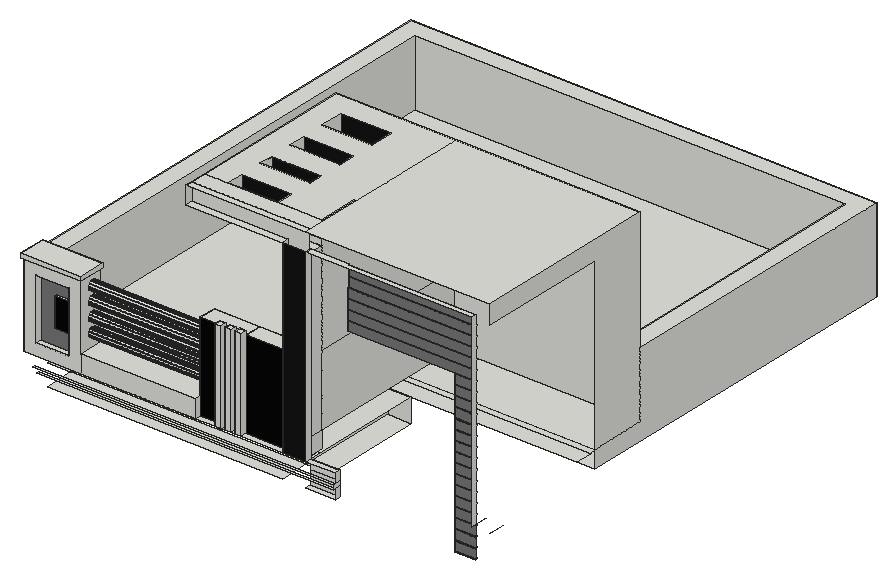
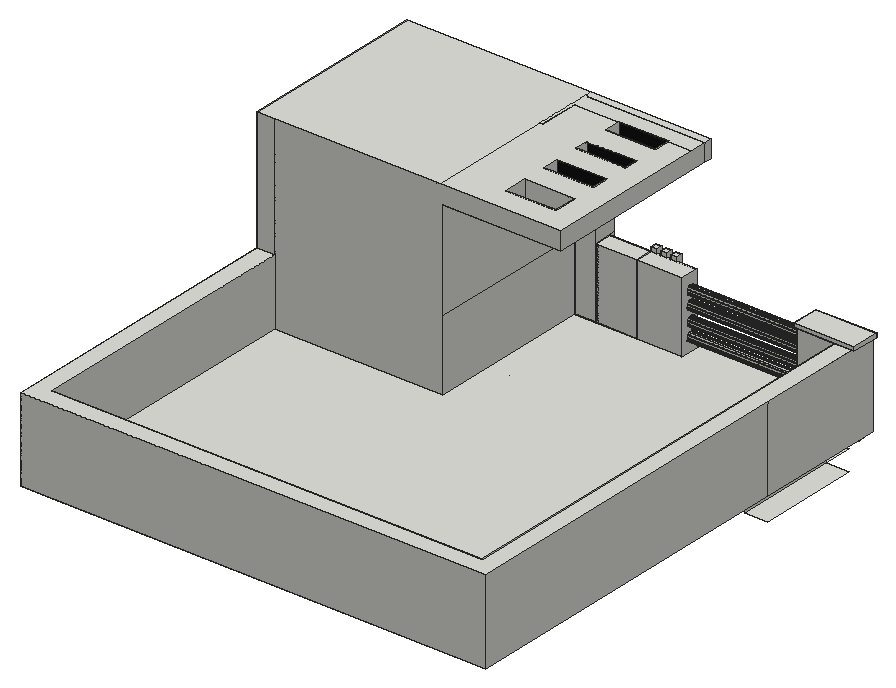
# SketchUp Ruby script. Lengths in inches.
U = 1.inch
M = Sketchup.active_model
def pt(a) = Geom::Point3d.new(a.map { |v| v * U })
def face(e, loops, mat)
  f = e.add_face(loops[0].map { |a| pt(a) })
  loops[1..].each { |l| e.add_face(l.map { |a| pt(a) }).erase! }
  f.material = f.back_material = mat if mat
  f
end
# faces: each face lists its corners as indices into pts; further lists are holes
def faces(e, pts, list, mat = nil) = list.each { |f| face(e, (f[0].is_a?(Array) ? f : [f]).map { |l| l.map { |i| pts[i] } }, mat) }
# xy, xz, yz: faces in a plane at the given z, y or x. An outline is a flat list of corners, or four numbers for a rectangle; further outlines are holes
def ring(l) = l.size == 4 ? [[l[0], l[1]], [l[2], l[1]], [l[2], l[3]], [l[0], l[3]]] : l.each_slice(2).to_a
def flat(e, list, mat, &to3) = list.each { |f| face(e, (f[0].is_a?(Array) ? f : [f]).map { |l| ring(l).map { |u, v| to3.(u, v) } }, mat) }
def xy(e, z, list, mat = nil) = flat(e, list, mat) { |x, y| [x, y, z] }
def xz(e, y, list, mat = nil) = flat(e, list, mat) { |x, z| [x, y, z] }
def yz(e, x, list, mat = nil) = flat(e, list, mat) { |y, z| [x, y, z] }
def lines(e, pts, list) = list.each { |a, b| e.add_line(pt(pts[a]), pt(pts[b])) }
# prism: a flat outline (further loops are holes) pulled along v
def prism(e, loops, v, mat = nil)
  f = face(e, loops, mat); d = Geom::Vector3d.new(v.map { |x| x * U })
  f.pushpull(f.normal.samedirection?(d) ? d.length : -d.length)
end
def box(e, o, s, mat = nil) = prism(e, [[o, [o[0] + s[0], o[1], o[2]], [o[0] + s[0], o[1] + s[1], o[2]], [o[0], o[1] + s[1], o[2]]]], [0, 0, s[2]], mat)
def at(x, y, z, deg = 0) = Geom::Transformation.translation(pt([x, y, z])) * Geom::Transformation.rotation(ORIGIN, Z_AXIS, deg.degrees)
def axes(o, x, y, z) = Geom::Transformation.new([*x, 0, *y, 0, *z, 0, *pt(o).to_a, 1])
def part(name) = M.definitions.add(name)
# library, detail: a bought-in or finely detailed component or shape, given as its bounding box
def library(name, o, s) = part(name).tap { |d| box(d.entities, o, s) }
def detail(e, o, s) = box(e.add_group.entities, o, s)
def put(e, d, t, mat = nil) = e.add_instance(d, t).tap { |i| i.material = mat if mat }
def group(e, t, mat = nil) = e.add_group.tap { |g| g.transformation = t; g.material = mat if mat }.entities
root = M.entities
M.materials.add("[0135_DarkGray]1").color = [119, 119, 119]
M.materials.add("[0136_Charcoal]").color = [7, 7, 7]
M.materials.add("[0136_Charcoal]1").color = [20, 20, 20]
xy(root,232.85,[[219.1875,3.625,229.75,4.125]])
xy(root,233.35,[[219.1875,3.625,229.75,4.125]])
xy(root,237,[[13,1.125,133.04,16.125],[145.04,1.125,160.04,4.125],[133.04,16.125,145.04,68.1875]])
xy(root,237.0625,[[1,16.125,12.875,68.1875]])
xy(root,237.93,[[219.1875,3.625,229.75,4.125]])
xy(root,238.43,[[219.1875,3.625,229.75,4.125]])
xy(root,242,[[8.5,0.125,160.04,1.125]])
xy(root,243,[[219.1875,3.625,229.75,4.125]])
xy(root,243.5,[[219.1875,3.625,229.75,4.125]])
xy(root,244,[[6.5,0.125,160.04,1.125]])
xy(root,248.08,[[219.1875,3.625,229.75,4.125]])
xy(root,248.58,[[219.1875,3.625,229.75,4.125]])
xy(root,249,[[1,1.125,12.875,68.1875],[12.875,1.125,12.875,16.125,133.04,16.125,133.04,13.125,111.875,13.125,111.875,1.125,108.875,1.125,108.875,4.125,106.8125,4.125,106.8125,1.125,103.8125,1.125,103.8125,4.125,101.6875,4.125,101.6875,1.125,98.6875,1.125,98.6875,4.125,88.625,4.125,88.625,1.125],[88.625,1.125,98.6875,4.125],[101.6875,1.125,103.8125,4.125],[106.8125,1.125,108.875,4.125],
  [111.875,1.125,133.04,4.125],[133.04,1.125,143.7,10.125],[145.04,1.125,160.04,4.125],[111.875,4.125,133.04,13.125],[145.04,4.125,143.7,4.87,143.7,10.125,145.04,10.125],
  [133.04,10.125,143.7,13.125],[143.7,10.125,143.7,13.125,133.04,13.125,133.04,68.1875,145.04,68.1875,145.04,10.125],[12.875,16.125,133.04,68.1875],[1,68.1875,229.75,68.1875,229.75,77.1875,10,77.1875,10,239.1875,229.75,239.1875,229.75,248.1875,1,248.1875],[229.75,68.1875,238.75,248.1875],
  [10,77.1875,229.75,239.1875]])
xy(root,253.15,[[219.1875,3.625,229.75,4.125]])
xy(root,253.65,[[219.1875,3.625,229.75,4.125]])
xy(root,255,[[7,1.125,24,4.125]])
xy(root,258,[[30,1.125,88.625,1.125,88.625,13.125,143.7,13.125,143.7,97.125,229.75,97.125,229.75,239.1875,10,239.1875,10,13.125,30,13.125]])
xy(root,258.23,[[219.1875,3.625,229.75,4.125]])
xy(root,258.73,[[219.1875,3.625,229.75,4.125]])
xy(root,263.3,[[219.1875,3.625,229.75,4.125]])
xy(root,263.8,[[219.1875,3.625,229.75,4.125]])
xy(root,264,[[15.5,2.625,24,4.125]])
xy(root,268.375,[[219.1875,3.625,229.75,4.125]])
xy(root,268.875,[[219.1875,3.625,229.75,4.125]])
xy(root,273.45,[[219.1875,3.625,229.75,4.125]])
xy(root,273.95,[[219.1875,3.625,229.75,4.125]])
xy(root,278.53,[[219.1875,3.625,229.75,4.125]])
xy(root,278.5625,[[15.5,2.625,24,4.125]])
xy(root,279.03,[[219.1875,3.625,229.75,4.125]])
xy(root,283.6,[[219.1875,3.625,229.75,4.125]])
xy(root,284.1,[[219.1875,3.625,229.75,4.125]])
xy(root,286,[[7,1.125,24,4.125]])
xy(root,288.68,[[219.1875,3.625,229.75,4.125]])
xy(root,289.18,[[219.1875,3.625,229.75,4.125]])
xy(root,292,[[0,0,31,1.125],[0,1.125,1,13.125],[1,1.125,30,13.125],[30,1.125,31,4.125],[30,4.125,31,14.125],
  [0,13.125,1,14.125],[1,13.125,10,14.125],[10,13.125,30,14.125],[1,14.125,10,14.125,10,239.1875,229.75,239.1875,229.75,97.125,238.75,97.125,238.75,248.1875,1,248.1875]])
xy(root,293.75,[[219.1875,3.625,229.75,4.125]])
xy(root,294,[[0,0,31,14.125],[88.625,4.125,111.875,13.125],[111.875,4.125,132.95,13.125]])
xy(root,294.25,[[219.1875,3.625,229.75,4.125]])
xy(root,296,[[98.6875,1.125,101.6875,4.125],[103.8125,1.125,106.8125,4.125],[108.875,1.125,111.875,4.125]])
xy(root,298.83,[[219.1875,3.625,229.75,4.125]])
xy(root,299.33,[[219.1875,3.625,229.75,4.125]])
xy(root,303.9,[[219.1875,3.625,229.75,4.125]])
xy(root,304.4,[[219.1875,3.625,229.75,4.125]])
xy(root,308.98,[[219.1875,3.625,229.75,4.125]])
xy(root,309.48,[[219.1875,3.625,229.75,4.125]])
xy(root,314.05,[[219.1875,3.625,229.75,4.125]])
xy(root,314.55,[[164.62,3.625,229.75,4.125]])
xy(root,319.125,[[164.62,3.625,229.75,4.125]])
xy(root,319.625,[[164.62,3.625,229.75,4.125]])
xy(root,324.2,[[164.62,3.625,229.75,4.125]])
xy(root,324.7,[[164.62,3.625,229.75,4.125]])
xy(root,329.28,[[164.62,3.625,229.75,4.125]])
xy(root,329.78,[[164.62,3.625,229.75,4.125]])
xy(root,334.35,[[164.62,3.625,229.75,4.125]])
xy(root,334.85,[[164.62,3.6875,229.75,4.125]])
xy(root,339.43,[[164.62,3.6875,229.75,4.125]])
xy(root,339.93,[[164.62,3.6875,229.75,4.125]])
xy(root,342,[[132.95,4.87,143.7,13.125]])
xy(root,345,[[83.7,1.125,132.95,4.87],[145.04,1.125,145.04,4.125,164.62,4.125,164.62,3.6875,229.75,3.6875,229.75,1.125],[[83.7,4.87,83.7,97.125,143.7,97.125,143.7,13.125,132.95,13.125,132.95,4.87],[95.7,13.125,121.04,85.125]]])
xy(root,345,[[95.7,21.5625,121.04,33.5625],[95.7,40.66,121.04,52.66],[95.7,61.125,121.04,73.125]],"[0136_Charcoal]1")
xy(root,354,[[83.7,1.125,145.04,1.125,145.04,4.125,143.7,4.87,83.7,4.87],[145.04,1.125,238.75,97.125],[145.04,4.125,145.04,33.5625,143.7,33.5625,143.7,13.125,83.7,13.125,83.7,4.87,143.7,4.87],[[83.7,13.125,95.7,13.125,95.7,21.5625,121.04,21.5625,121.04,13.125,143.7,13.125,143.7,33.5625,145.04,33.5625,145.04,97.125,83.7,97.125],[95.7,73.125,121.04,85.125],[95.7,52.66,121.04,61.125],[95.7,33.5625,121.04,40.66]]])
xz(root,0,[[0,292,31,294]])
xz(root,1.125,[[[1,249,30,292],[7,255,24,286]],[30,249,88.625,258],[98.6875,249,101.6875,296],[103.8125,249,106.8125,296],[108.875,249,111.875,296]])
xz(root,1.125,[[133.04,249,145.04,249,145.04,345,132.95,345,132.95,294]],"[0136_Charcoal]1")
xz(root,2.625,[[15.5,264,24,278.5625]],"[0136_Charcoal]")
xz(root,3.625,[[219.1875,233.35,229.75,237.93],[219.1875,238.43,229.75,243],[219.1875,243.5,229.75,248.08],[219.1875,248.58,229.75,253.15],[219.1875,253.65,229.75,258.23],
  [219.1875,258.73,229.75,263.3],[219.1875,263.8,229.75,268.375],[219.1875,268.875,229.75,273.45],[219.1875,273.95,229.75,278.53],[219.1875,279.03,229.75,283.6],
  [219.1875,284.1,229.75,288.68],[219.1875,289.18,229.75,293.75],[219.1875,294.25,229.75,298.83],[219.1875,299.33,229.75,303.9],[219.1875,304.4,229.75,308.98],
  [219.1875,309.48,229.75,314.05],[164.62,314.55,229.75,319.125],[164.62,319.625,229.75,324.2],[164.62,324.7,229.75,329.28],[164.62,329.78,229.75,334.35]],"[0135_DarkGray]1")
xz(root,3.6875,[[164.62,334.85,229.75,339.43],[164.62,339.93,229.75,345]],"[0135_DarkGray]1")
xz(root,4.125,[[219.1875,232.85,229.75,233.35],[145.04,237,160.04,242],[219.1875,237.93,229.75,238.43],[145.04,242,160.04,244],[219.1875,243,229.75,243.5],
  [145.04,244,160.04,249],[219.1875,248.08,229.75,248.58],[132.95,249,133.04,249,132.95,294],[219.1875,253.15,229.75,253.65],[219.1875,258.23,229.75,258.73],
  [219.1875,263.3,229.75,263.8],[219.1875,268.375,229.75,268.875],[219.1875,273.45,229.75,273.95],[219.1875,278.53,229.75,279.03],[219.1875,283.6,229.75,284.1],
  [219.1875,288.68,229.75,289.18],[219.1875,293.75,229.75,294.25],[98.6875,294,101.6875,296],[103.8125,294,106.8125,296],[108.875,294,111.875,296],
  [219.1875,298.83,229.75,299.33],[219.1875,303.9,229.75,304.4],[219.1875,308.98,229.75,309.48],[219.1875,314.05,229.75,314.55],[164.62,319.125,219.1875,319.625],
  [219.1875,319.125,229.75,319.625],[164.62,324.2,219.1875,324.7],[219.1875,324.2,229.75,324.7],[164.62,329.28,219.1875,329.78],[219.1875,329.28,229.75,329.78],
  [164.62,334.35,219.1875,334.85],[219.1875,334.35,229.75,334.85],[164.62,339.43,219.1875,339.93],[219.1875,339.43,229.75,339.93]])
xz(root,4.125,[[7,255,24,255,24,264,15.5,264,15.5,278.5625,24,278.5625,24,286,7,286]],"[0135_DarkGray]1")
xz(root,4.125,[[88.625,249,98.6875,294],[101.6875,249,103.8125,294],[106.8125,249,108.875,294],[111.875,249,132.95,294]],"[0136_Charcoal]")
xz(root,4.87,[[132.95,342,143.7,342,143.7,354,83.7,354,83.7,345,132.95,345]])
xz(root,13.125,[[111.875,249,111.875,258,133.02,258,133.04,249],[133.04,249,133.02,258,143.7,258,143.7,249],[10,258,30,292],[88.625,258,111.875,294],[111.875,258,131.96,294],
  [131.96,258,131.96,294,132.95,294,133.02,258],[133.02,258,132.95,294,132.95,342,143.7,342,143.7,258],[132.95,342,133.04,345],[133.04,342,143.7,345]])
xz(root,13.125,[[95.7,345,121.04,354]],"[0136_Charcoal]1")
xz(root,14.125,[[0,292,31,294]])
xz(root,21.5625,[[95.7,345,121.04,354]],"[0136_Charcoal]1")
xz(root,33.5625,[[95.7,345,121.04,354]],"[0136_Charcoal]1")
xz(root,40.66,[[95.7,345,121.04,354]],"[0136_Charcoal]1")
xz(root,52.66,[[95.7,345,121.04,354]],"[0136_Charcoal]1")
xz(root,61.125,[[95.7,345,121.04,354]],"[0136_Charcoal]1")
xz(root,68.1875,[[133.04,237,145.04,249]])
xz(root,73.125,[[95.7,345,121.04,354]])
xz(root,85.125,[[95.7,345,121.04,354]],"[0136_Charcoal]1")
xz(root,97.125,[[143.7,258,143.7,345,83.7,345,83.7,354,229.75,354,229.75,258],[229.75,292,238.75,354]])
xz(root,239.1875,[[10,258,229.75,292]])
xz(root,248.1875,[[1,249,238.75,292]])
yz(root,0,[[0,292,14.125,294]])
yz(root,1,[[1.125,249,68.1875,292],[68.1875,249,248.1875,292]])
yz(root,7,[[1.125,255,4.125,286]])
yz(root,10,[[13.125,258,239.1875,292]])
yz(root,12.875,[[16.125,237.0625,68.1875,249]])
yz(root,15.5,[[2.625,264,4.125,278.5625]])
yz(root,24,[[1.125,255,4.125,264],[1.125,264,2.625,278.5625],[1.125,278.5625,4.125,286]])
yz(root,30,[[[1.125,258,13.125,292],[8.14,269.95,7.52,270.03,6.95,270.27,6.46,270.64,6.08,271.14,5.84,271.71,5.76,272.32,5.84,272.9375,6.08,273.51,6.46,274,6.95,274.38,7.52,274.62,8.14,274.7,8.75,274.62,9.32,274.38,9.82,274,10.19,273.51,10.43,272.9375,10.51,272.32,10.43,271.71,10.19,271.14,9.82,270.64,9.32,270.27,8.75,270.03],[8.14,277.26,7.52,277.34,6.95,277.58,6.46,277.96,6.08,278.45,5.84,279.02,5.76,279.64,5.84,280.25,6.08,280.82,6.46,281.32,6.95,281.69,7.52,281.93,8.14,282.01,8.75,281.93,9.32,281.69,9.82,281.32,10.19,280.82,10.43,280.25,10.51,279.64,10.43,279.02,10.19,278.45,9.82,277.96,9.32,277.58,8.75,277.34],[8.14,284.2,7.52,284.28,6.95,284.52,6.46,284.89,6.08,285.39,5.84,285.96,5.76,286.57,5.84,287.1875,6.08,287.76,6.46,288.25,6.95,288.63,7.52,288.87,8.14,288.95,8.75,288.87,9.32,288.63,9.82,288.25,10.19,287.76,10.43,287.1875,10.51,286.57,10.43,285.96,10.19,285.39,9.82,284.89,9.32,284.52,8.75,284.28],[8.14,262.89,7.52,262.97,6.95,263.2,6.46,263.58,6.08,264.07,5.84,264.65,5.76,265.26,5.84,265.875,6.08,266.45,6.46,266.94,6.95,267.32,7.52,267.55,8.14,267.64,8.75,267.55,9.32,267.32,9.82,266.94,10.19,266.45,10.43,265.875,10.51,265.26,10.43,264.65,10.19,264.07,9.82,263.58,9.32,263.2,8.75,262.97]]])
yz(root,31,[[0,292,14.125,294]])
yz(root,83.7,[[1.125,345,4.87,354],[4.87,345,97.125,354]])
yz(root,88.625,[[1.125,249,4.125,258],[[4.125,258,13.125,294],[8.14,284.2,8.75,284.28,9.32,284.52,9.82,284.89,10.19,285.39,10.43,285.96,10.51,286.57,10.43,287.1875,10.19,287.76,9.82,288.25,9.32,288.63,8.75,288.87,8.14,288.95,7.52,288.87,6.95,288.63,6.46,288.25,6.08,287.76,5.84,287.1875,5.76,286.57,5.84,285.96,6.08,285.39,6.46,284.89,6.95,284.52,7.52,284.28],[8.14,277.26,8.75,277.34,9.32,277.58,9.82,277.96,10.19,278.45,10.43,279.02,10.51,279.64,10.43,280.25,10.19,280.82,9.82,281.32,9.32,281.69,8.75,281.93,8.14,282.01,7.52,281.93,6.95,281.69,6.46,281.32,6.08,280.82,5.84,280.25,5.76,279.64,5.84,279.02,6.08,278.45,6.46,277.96,6.95,277.58,7.52,277.34]]])
yz(root,88.875,[[8.14,269.95,8.75,270.03,9.32,270.27,9.82,270.64,10.19,271.14,10.43,271.71,10.51,272.32,10.43,272.9375,10.19,273.51,9.82,274,9.32,274.38,8.75,274.62,8.14,274.7,7.52,274.62,6.95,274.38,6.46,274,6.08,273.51,5.84,272.9375,5.76,272.32,5.84,271.71,6.08,271.14,6.46,270.64,6.95,270.27,7.52,270.03]])
yz(root,88.9375,[[8.14,262.89,8.75,262.97,9.32,263.2,9.82,263.58,10.19,264.07,10.43,264.65,10.51,265.26,10.43,265.875,10.19,266.45,9.82,266.94,9.32,267.32,8.75,267.55,8.14,267.64,7.52,267.55,6.95,267.32,6.46,266.94,6.08,266.45,5.84,265.875,5.76,265.26,5.84,264.65,6.08,264.07,6.46,263.58,6.95,263.2,7.52,262.97]])
yz(root,95.7,[[13.125,345,21.5625,354],[33.5625,345,40.66,354],[52.66,345,61.125,354],[73.125,345,85.125,354]])
yz(root,98.6875,[[1.125,249,4.125,296]])
yz(root,101.6875,[[1.125,249,4.125,296]])
yz(root,103.8125,[[1.125,249,4.125,296]])
yz(root,106.8125,[[1.125,249,4.125,296]])
yz(root,108.875,[[1.125,249,4.125,296]])
yz(root,111.875,[[1.125,249,4.125,296],[4.125,249,13.125,294]])
yz(root,121.04,[[13.125,345,21.5625,354],[33.5625,345,40.66,354],[52.66,345,61.125,354],[73.125,345,85.125,354]])
yz(root,132.95,[[1.125,294,13.125,342],[1.125,342,4.87,345],[4.87,342,13.125,345]])
yz(root,133.04,[[16.125,237,68.1875,249]])
yz(root,143.7,[[4.87,249,13.125,258],[4.87,258,13.125,342],[13.125,258,97.125,294],[13.125,294,97.125,345],[13.125,345,33.5625,354]])
yz(root,145.04,[[1.125,249,4.125,345]])
yz(root,160.04,[[1.125,237,4.125,242],[0.125,242,4.125,244],[1.125,244,4.125,249]])
yz(root,164.62,[[3.625,314.55,4.125,319.125],[3.625,319.625,4.125,324.2],[3.625,324.7,4.125,329.28],[3.625,329.78,4.125,334.35],[3.6875,334.85,4.125,339.43],
  [3.6875,339.93,4.125,345]])
yz(root,219.1875,[[3.625,233.35,4.125,237.93],[3.625,238.43,4.125,243],[3.625,243.5,4.125,248.08],[3.625,248.58,4.125,253.15],[3.625,253.65,4.125,258.23],
  [3.625,258.73,4.125,263.3],[3.625,263.8,4.125,268.375],[3.625,268.875,4.125,273.45],[3.625,273.95,4.125,278.53],[3.625,279.03,4.125,283.6],
  [3.625,284.1,4.125,288.68],[3.625,289.18,4.125,293.75],[3.625,294.25,4.125,298.83],[3.625,299.33,4.125,303.9],[3.625,304.4,4.125,308.98],
  [3.625,309.48,4.125,314.05]])
yz(root,229.75,[[1.125,249,1.125,345,3.6875,345,3.6875,339.93,4.125,339.93,4.125,339.43,3.6875,339.43,3.6875,334.85,4.125,334.85,4.125,334.35,3.625,334.35,3.625,329.78,4.125,329.78,4.125,329.28,3.625,329.28,3.625,324.7,4.125,324.7,4.125,324.2,3.625,324.2,3.625,319.625,4.125,319.625,4.125,319.125,3.625,319.125,3.625,314.55,4.125,314.55,4.125,314.05,3.625,314.05,3.625,309.48,4.125,309.48,4.125,308.98,3.625,308.98,3.625,304.4,4.125,304.4,4.125,303.9,3.625,303.9,3.625,299.33,4.125,299.33,4.125,298.83,3.625,298.83,3.625,294.25,4.125,294.25,4.125,293.75,3.625,293.75,3.625,289.18,4.125,289.18,4.125,288.68,3.625,288.68,3.625,284.1,4.125,284.1,4.125,283.6,3.625,283.6,3.625,279.03,4.125,279.03,4.125,278.53,3.625,278.53,3.625,273.95,4.125,273.95,4.125,273.45,3.625,273.45,3.625,268.875,4.125,268.875,4.125,268.375,3.625,268.375,3.625,263.8,4.125,263.8,4.125,263.3,3.625,263.3,3.625,258.73,4.125,258.73,4.125,258.23,3.625,258.23,3.625,253.65,4.125,253.65,4.125,253.15,3.625,253.15,3.625,249],[97.125,258,239.1875,292]])
yz(root,238.75,[[68.1875,249,248.1875,249,248.1875,292,97.125,292,97.125,258,68.1875,258],[68.1875,258,97.125,258,97.125,354,1.125,354,1.125,344.33,68.1875,344.33]])
p = [[132.95,4.125,294],[133.04,4.125,249],[133.04,1.125,249],[132.95,1.125,294],[133.04,10.125,249],[133.04,13.125,249],
  [133.02,13.125,258],[132.95,13.125,294],[30,7.52,262.97],[30,8.14,262.89],[88.9375,8.14,262.89],[88.9375,7.52,262.97],
  [30,8.75,262.97],[88.9375,8.75,262.97],[30,6.95,263.2],[88.9375,6.95,263.2],[30,9.32,263.2],[88.9375,9.32,263.2],
  [30,6.46,263.58],[88.9375,6.46,263.58],[30,9.82,263.58],[88.9375,9.82,263.58],[30,6.08,264.07],[88.9375,6.08,264.07],
  [30,10.19,264.07],[88.9375,10.19,264.07],[30,5.84,264.65],[88.9375,5.84,264.65],[30,10.43,264.65],[88.9375,10.43,264.65],
  [30,5.76,265.26],[88.9375,5.76,265.26],[30,10.51,265.26],[88.9375,10.51,265.26],[30,5.84,265.875],[88.9375,5.84,265.875],
  [30,10.43,265.875],[88.9375,10.43,265.875],[30,6.08,266.45],[88.9375,6.08,266.45],[30,10.19,266.45],[88.9375,10.19,266.45],
  [30,6.46,266.94],[88.9375,6.46,266.94],[30,9.82,266.94],[88.9375,9.82,266.94],[30,6.95,267.32],[88.9375,6.95,267.32],
  [30,9.32,267.32],[88.9375,9.32,267.32],[30,7.52,267.55],[88.9375,7.52,267.55],[30,8.75,267.55],[88.9375,8.75,267.55],
  [30,8.14,267.64],[88.9375,8.14,267.64],[30,7.52,270.03],[30,8.14,269.95],[88.875,8.14,269.95],[88.875,7.52,270.03],
  [30,8.75,270.03],[88.875,8.75,270.03],[30,6.95,270.27],[88.875,6.95,270.27],[30,9.32,270.27],[88.875,9.32,270.27],
  [30,6.46,270.64],[88.875,6.46,270.64],[30,9.82,270.64],[88.875,9.82,270.64],[30,6.08,271.14],[88.875,6.08,271.14],
  [30,10.19,271.14],[88.875,10.19,271.14],[30,5.84,271.71],[88.875,5.84,271.71],[30,10.43,271.71],[88.875,10.43,271.71],
  [30,5.76,272.32],[88.875,5.76,272.32],[30,10.51,272.32],[88.875,10.51,272.32],[30,5.84,272.9375],[88.875,5.84,272.9375],
  [30,10.43,272.9375],[88.875,10.43,272.9375],[30,6.08,273.51],[88.875,6.08,273.51],[30,10.19,273.51],[88.875,10.19,273.51],
  [30,6.46,274],[88.875,6.46,274],[30,9.82,274],[88.875,9.82,274],[30,6.95,274.38],[88.875,6.95,274.38],
  [30,9.32,274.38],[88.875,9.32,274.38],[30,7.52,274.62],[88.875,7.52,274.62],[30,8.75,274.62],[88.875,8.75,274.62],
  [30,8.14,274.7],[88.875,8.14,274.7],[30,6.95,277.58],[30,7.52,277.34],[88.625,7.52,277.34],[88.625,6.95,277.58],
  [30,8.14,277.26],[88.625,8.14,277.26],[30,8.75,277.34],[88.625,8.75,277.34],[30,9.32,277.58],[88.625,9.32,277.58],
  [30,6.46,277.96],[88.625,6.46,277.96],[30,9.82,277.96],[88.625,9.82,277.96],[30,6.08,278.45],[88.625,6.08,278.45],
  [30,10.19,278.45],[88.625,10.19,278.45],[30,5.84,279.02],[88.625,5.84,279.02],[30,10.43,279.02],[88.625,10.43,279.02],
  [30,5.76,279.64],[88.625,5.76,279.64],[30,10.51,279.64],[88.625,10.51,279.64],[30,5.84,280.25],[88.625,5.84,280.25],
  [30,10.43,280.25],[88.625,10.43,280.25],[30,6.08,280.82],[88.625,6.08,280.82],[30,10.19,280.82],[88.625,10.19,280.82],
  [30,6.46,281.32],[88.625,6.46,281.32],[30,9.82,281.32],[88.625,9.82,281.32],[30,6.95,281.69],[88.625,6.95,281.69],
  [30,9.32,281.69],[88.625,9.32,281.69],[30,7.52,281.93],[88.625,7.52,281.93],[30,8.75,281.93],[88.625,8.75,281.93],
  [30,8.14,282.01],[88.625,8.14,282.01],[30,7.52,284.28],[30,8.14,284.2],[88.625,8.14,284.2],[88.625,7.52,284.28],
  [30,8.75,284.28],[88.625,8.75,284.28],[30,6.95,284.52],[88.625,6.95,284.52],[30,9.32,284.52],[88.625,9.32,284.52],
  [30,6.46,284.89],[88.625,6.46,284.89],[30,9.82,284.89],[88.625,9.82,284.89],[30,6.08,285.39],[88.625,6.08,285.39],
  [30,10.19,285.39],[88.625,10.19,285.39],[30,5.84,285.96],[88.625,5.84,285.96],[30,10.43,285.96],[88.625,10.43,285.96],
  [30,5.76,286.57],[88.625,5.76,286.57],[30,10.51,286.57],[88.625,10.51,286.57],[30,5.84,287.1875],[88.625,5.84,287.1875],
  [30,10.43,287.1875],[88.625,10.43,287.1875],[30,6.08,287.76],[88.625,6.08,287.76],[30,10.19,287.76],[88.625,10.19,287.76],
  [30,6.46,288.25],[88.625,6.46,288.25],[30,9.82,288.25],[88.625,9.82,288.25],[30,6.95,288.63],[88.625,6.95,288.63],
  [30,9.32,288.63],[88.625,9.32,288.63],[30,7.52,288.87],[88.625,7.52,288.87],[30,8.75,288.87],[88.625,8.75,288.87],
  [30,8.14,288.95],[88.625,8.14,288.95],[143.7,4.125,342],[143.7,4.87,342],[238.75,10.125,249],[238.75,1.125,249],
  [133.04,68.1875,249],[133.04,68.1875,258],[133.04,68.1875,344.33],[133.04,13.125,344.33],[238.75,68.1875,258],[143.7,68.1875,258],
  [238.75,68.1875,344.33],[229.75,10.125,249],[229.75,4.125,249],[133.04,10.125,344.33],[145.04,16.125,237],[145.04,10.125,237]]
faces(root,p,[[0,1,2,3],[0,1,4,5,6,7],[8,9,10,11],[9,12,13,10],[14,8,11,15],[12,16,17,13],[18,14,15,19],[16,20,21,17],
  [22,18,19,23],[20,24,25,21],[26,22,23,27],[24,28,29,25],[30,26,27,31],[28,32,33,29],[34,30,31,35],[32,36,37,33],
  [38,34,35,39],[36,40,41,37],[42,38,39,43],[40,44,45,41],[46,42,43,47],[44,48,49,45],[50,46,47,51],[48,52,53,49],
  [54,50,51,55],[52,54,55,53],[56,57,58,59],[57,60,61,58],[62,56,59,63],[60,64,65,61],[66,62,63,67],[64,68,69,65],
  [70,66,67,71],[68,72,73,69],[74,70,71,75],[72,76,77,73],[78,74,75,79],[76,80,81,77],[82,78,79,83],[80,84,85,81],
  [86,82,83,87],[84,88,89,85],[90,86,87,91],[88,92,93,89],[94,90,91,95],[92,96,97,93],[98,94,95,99],[96,100,101,97],
  [102,98,99,103],[100,102,103,101],[104,105,106,107],[105,108,109,106],[108,110,111,109],[110,112,113,111],[114,104,107,115],[112,116,117,113],
  [118,114,115,119],[116,120,121,117],[122,118,119,123],[120,124,125,121],[126,122,123,127],[124,128,129,125],[130,126,127,131],[128,132,133,129],
  [134,130,131,135],[132,136,137,133],[138,134,135,139],[136,140,141,137],[142,138,139,143],[140,144,145,141],[146,142,143,147],[144,148,149,145],
  [150,146,147,151],[148,150,151,149],[152,153,154,155],[153,156,157,154],[158,152,155,159],[156,160,161,157],[162,158,159,163],[160,164,165,161],
  [166,162,163,167],[164,168,169,165],[170,166,167,171],[168,172,173,169],[174,170,171,175],[172,176,177,173],[178,174,175,179],[176,180,181,177],
  [182,178,179,183],[180,184,185,181],[186,182,183,187],[184,188,189,185],[190,186,187,191],[188,192,193,189],[194,190,191,195],[192,196,197,193],
  [198,194,195,199],[196,198,199,197]])
lines(root,p,[[200,201],[202,203],[204,205],[206,207],[208,209],[210,206],[211,212],[207,213],[214,215]])
